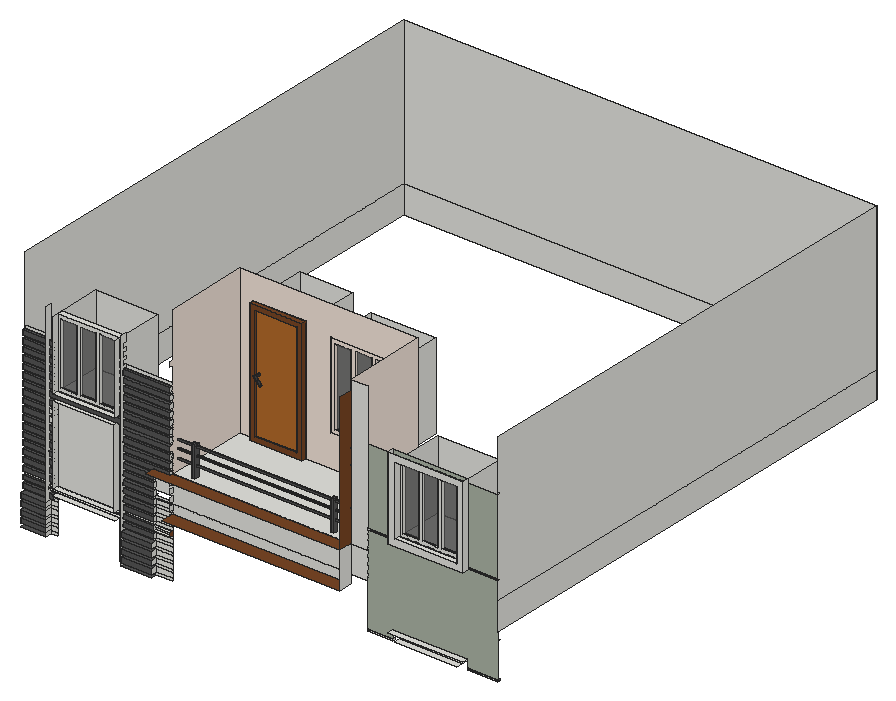
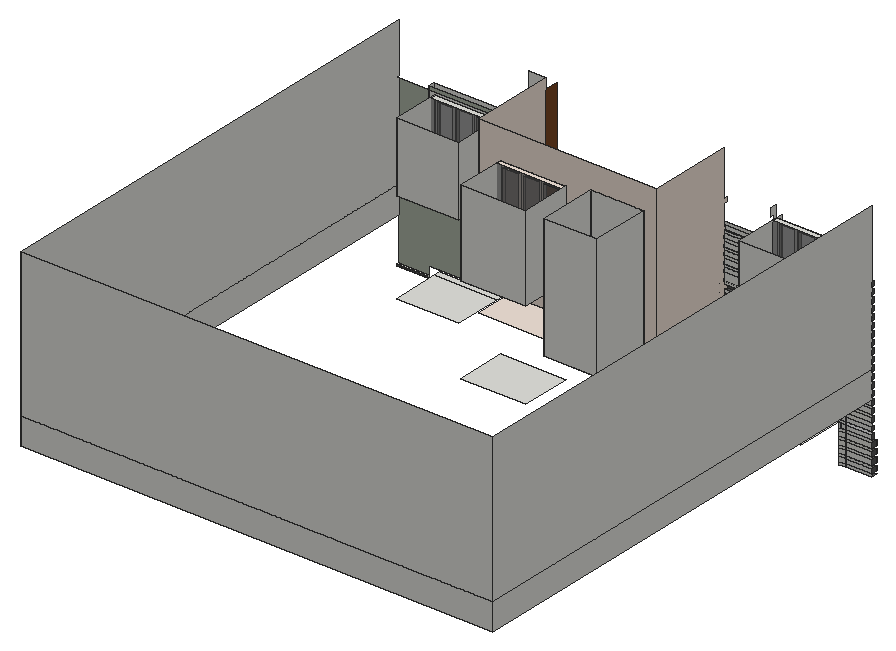
# SketchUp Ruby script. Lengths in inches.
U = 1.inch
M = Sketchup.active_model
def pt(a) = Geom::Point3d.new(a.map { |v| v * U })
def face(e, loops, mat)
  f = e.add_face(loops[0].map { |a| pt(a) })
  loops[1..].each { |l| e.add_face(l.map { |a| pt(a) }).erase! }
  f.material = f.back_material = mat if mat
  f
end
# faces: each face lists its corners as indices into pts; further lists are holes
def faces(e, pts, list, mat = nil) = list.each { |f| face(e, (f[0].is_a?(Array) ? f : [f]).map { |l| l.map { |i| pts[i] } }, mat) }
# xy, xz, yz: faces in a plane at the given z, y or x. An outline is a flat list of corners, or four numbers for a rectangle; further outlines are holes
def ring(l) = l.size == 4 ? [[l[0], l[1]], [l[2], l[1]], [l[2], l[3]], [l[0], l[3]]] : l.each_slice(2).to_a
def flat(e, list, mat, &to3) = list.each { |f| face(e, (f[0].is_a?(Array) ? f : [f]).map { |l| ring(l).map { |u, v| to3.(u, v) } }, mat) }
def xy(e, z, list, mat = nil) = flat(e, list, mat) { |x, y| [x, y, z] }
def xz(e, y, list, mat = nil) = flat(e, list, mat) { |x, z| [x, y, z] }
def yz(e, x, list, mat = nil) = flat(e, list, mat) { |y, z| [x, y, z] }
def lines(e, pts, list) = list.each { |a, b| e.add_line(pt(pts[a]), pt(pts[b])) }
# prism: a flat outline (further loops are holes) pulled along v
def prism(e, loops, v, mat = nil)
  f = face(e, loops, mat); d = Geom::Vector3d.new(v.map { |x| x * U })
  f.pushpull(f.normal.samedirection?(d) ? d.length : -d.length)
end
def box(e, o, s, mat = nil) = prism(e, [[o, [o[0] + s[0], o[1], o[2]], [o[0] + s[0], o[1] + s[1], o[2]], [o[0], o[1] + s[1], o[2]]]], [0, 0, s[2]], mat)
def at(x, y, z, deg = 0) = Geom::Transformation.translation(pt([x, y, z])) * Geom::Transformation.rotation(ORIGIN, Z_AXIS, deg.degrees)
def axes(o, x, y, z) = Geom::Transformation.new([*x, 0, *y, 0, *z, 0, *pt(o).to_a, 1])
def part(name) = M.definitions.add(name)
# library, detail: a bought-in or finely detailed component or shape, given as its bounding box
def library(name, o, s) = part(name).tap { |d| box(d.entities, o, s) }
def detail(e, o, s) = box(e.add_group.entities, o, s)
def put(e, d, t, mat = nil) = e.add_instance(d, t).tap { |i| i.material = mat if mat }
def group(e, t, mat = nil) = e.add_group.tap { |g| g.transformation = t; g.material = mat if mat }.entities
root = M.entities
M.materials.add("Generic\#1").color = [85, 85, 85]
M.materials.add("Generic\#2").color = [170, 178, 163]
M.materials.add("Generic\#4").color = [241, 227, 216]
M.materials.add("[Color M00]").color = [255, 255, 255]
M.materials.add("[Color M07]").color = [58, 58, 58]
M.materials.add("[Translucent Glass Gray]").color = [91, 91, 91]
M.materials["[Translucent Glass Gray]"].alpha = 0.55
M.materials.add("[Wood Bamboo]").color = [177, 105, 43]
M.materials.add("[Wood Veneer 01]").color = [120, 70, 37]
c1 = part("Group\#3")
xy(c1.entities,0,[[0,4.93,60.125,10.18]])
xy(c1.entities,5.66,[[5.66,4.93,54.46,7.18]],"[Wood Veneer 01]")
xy(c1.entities,68.44,[[8.18,1.47,8.18,7.18,9.93,7.18,9.93,2.62]],"[Color M07]")
xy(c1.entities,70.41,[[8.19,0,9.94,1.15,9.94,7.18,8.19,7.18]],"[Color M07]")
xy(c1.entities,134.78,[[5.66,4.93,54.46,7.18]])
xy(c1.entities,140.4375,[[0,4.93,60.125,10.18]],"[Wood Veneer 01]")
xz(c1.entities,4.93,[[[0,0,60.125,140.4375],[5.66,5.66,54.46,134.78]]],"[Wood Veneer 01]")
xz(c1.entities,7.18,[[[5.66,5.66,54.46,134.78],[8.18,68.44,8.19,70.41,9.94,70.41,9.93,68.44]],[8.18,68.44,8.19,70.41,9.94,70.41,9.93,68.44]],"[Wood Bamboo]")
xz(c1.entities,10.18,[[0,0,60.125,140.4375]])
yz(c1.entities,0,[[4.93,0,10.18,140.4375]],"[Wood Veneer 01]")
yz(c1.entities,5.66,[[4.93,5.66,7.18,134.78]],"[Wood Veneer 01]")
yz(c1.entities,54.46,[[4.93,5.66,7.18,134.78]],"[Wood Veneer 01]")
yz(c1.entities,60.125,[[4.93,0,10.18,140.4375]],"[Wood Veneer 01]")
p = [[8.19,0,70.41],[8.18,1.47,68.44],[14.45,1.47,61.21],[15.43,0,62.06],[15.45,2.62,62.07],[16.43,1.15,62.92],
  [9.93,2.62,68.44],[9.94,1.15,70.41],[8.19,7.18,70.41],[8.18,7.18,68.44],[9.93,7.18,68.44],[9.94,7.18,70.41],
  [8.95,0.93,69.83],[15.58,0.93,62.1875],[8.95,7.18,69.83]]
faces(c1.entities,p,[[0,1,2,3],[3,2,4,5],[1,6,4,2],[7,0,3,5],[6,7,5,4],[8,9,1,0],[10,11,7,6]],"[Color M07]")
lines(c1.entities,p,[[12,13],[14,12]])
c2 = part("Group\#1")
xy(c2.entities,0,[[0,0,70.8125,6.0625]])
xy(c2.entities,4.26,[[4.26,0,22.19,2.0625],[26.44,0,44.37,2.0625],[48.63,0,66.56,2.0625]])
xy(c2.entities,75.06,[[4.26,0,22.19,2.0625],[26.44,0,44.37,2.0625],[48.63,0,66.56,2.0625]])
xy(c2.entities,79.3125,[[0,0,70.8125,6.0625]])
xz(c2.entities,0,[[[0,0,70.8125,79.3125],[26.44,4.26,44.37,75.06],[4.26,4.26,22.19,75.06],[48.63,4.26,66.56,75.06]]])
xz(c2.entities,2.0625,[[4.26,4.26,22.19,75.06],[26.44,4.26,44.37,75.06],[48.63,4.26,66.56,75.06]],"[Translucent Glass Gray]")
xz(c2.entities,6.0625,[[0,0,70.8125,79.3125]],"[Translucent Glass Gray]")
yz(c2.entities,0,[[0,0,6.0625,79.3125]])
yz(c2.entities,4.26,[[0,4.26,2.0625,75.06]])
yz(c2.entities,22.19,[[0,4.26,2.0625,75.06]])
yz(c2.entities,26.44,[[0,4.26,2.0625,75.06]])
yz(c2.entities,44.37,[[0,4.26,2.0625,75.06]])
yz(c2.entities,48.63,[[0,4.26,2.0625,75.06]])
yz(c2.entities,66.56,[[0,4.26,2.0625,75.06]])
yz(c2.entities,70.8125,[[0,0,6.0625,79.3125]])
c3 = part("Group\#4")
xy(c3.entities,0,[[0,0,168,3.625]])
xy(c3.entities,5.375,[[0,0,168,3.625]])
xz(c3.entities,0,[[0,0,168,5.375]])
yz(c3.entities,0,[[0,0,3.625,5.375]])
c4 = part("Group\#2")
xy(c4.entities,0,[[0,0,74.5625,5.5]])
xy(c4.entities,4.83,[[4.83,0,23.24,2.5],[28.07,0,46.49,2.5],[51.32,0,69.73,2.5]])
xy(c4.entities,93.17,[[4.83,0,23.24,2.5],[28.07,0,46.49,2.5],[51.32,0,69.73,2.5]])
xy(c4.entities,98,[[0,0,74.5625,5.5]])
xz(c4.entities,0,[[[0,0,74.5625,98],[28.07,4.83,46.49,93.17],[51.32,4.83,69.73,93.17],[4.83,4.83,23.24,93.17]]])
xz(c4.entities,2.5,[[4.83,4.83,23.24,93.17],[28.07,4.83,46.49,93.17],[51.32,4.83,69.73,93.17]],"[Translucent Glass Gray]")
xz(c4.entities,5.5,[[0,0,74.5625,98]],"[Translucent Glass Gray]")
yz(c4.entities,0,[[0,0,5.5,98]])
yz(c4.entities,4.83,[[0,4.83,2.5,93.17]])
yz(c4.entities,23.24,[[0,4.83,2.5,93.17]])
yz(c4.entities,28.07,[[0,4.83,2.5,93.17]])
yz(c4.entities,46.49,[[0,4.83,2.5,93.17]])
yz(c4.entities,51.32,[[0,4.83,2.5,93.17]])
yz(c4.entities,69.73,[[0,4.83,2.5,93.17]])
yz(c4.entities,74.5625,[[0,0,5.5,98]])
xy(root,287.75,[[3.6875,24.0625,33.1875,31.0625],[118.35,24.0625,153.3125,31.0625]],"Generic\#1")
xy(root,291.0625,[[3.6875,24.0625,33.1875,31.0625],[118.35,24.0625,153.3125,31.0625]],"Generic\#1")
xy(root,296.4375,[[3.6875,24.0625,33.1875,31.0625],[118.35,24.0625,153.3125,31.0625]],"Generic\#1")
xy(root,299.75,[[3.6875,24.0625,33.1875,31.0625],[118.35,24.0625,153.3125,31.0625]],"Generic\#1")
xy(root,305.125,[[3.6875,24.0625,33.1875,31.0625],[118.35,24.0625,153.3125,31.0625]],"Generic\#1")
xy(root,308.4375,[[3.6875,24.0625,33.1875,31.0625],[118.35,24.0625,153.3125,31.0625]],"Generic\#1")
xy(root,313.8125,[[3.6875,24.0625,33.1875,31.0625],[118.35,24.0625,153.3125,31.0625]],"Generic\#1")
xy(root,315.5,[[395.4375,31.0625,423.8125,32.9375],[508.98,31.0625,543.6875,32.9375]])
xy(root,317.125,[[3.6875,24.0625,33.1875,31.0625],[118.35,24.0625,153.3125,31.0625]],"Generic\#1")
xy(root,317.5,[[395.4375,31.0625,423.8125,32.9375],[508.98,31.0625,543.6875,32.9375]])
xy(root,319.52,[[430.99,24.0625,501.8,31.0625],[430.99,31.0625,501.8,85.4375]])
xy(root,322.5,[[3.6875,24.0625,33.1875,31.0625],[118.35,24.0625,153.3125,31.0625]],"Generic\#1")
xy(root,325.8125,[[3.6875,27.4375,38.93,31.0625],[118.35,27.75,153.3125,31.0625]])
xy(root,326.69,[[423.8125,24.0625,508.98,31.0625]])
xy(root,331.1875,[[3.6875,27.4375,38.93,31.0625],[118.35,27.75,153.3125,31.0625]],"Generic\#1")
xy(root,331.7,[[40.36,24.0625,111.18,31.0625],[40.36,31.0625,111.18,85.4375]])
xy(root,333.91,[[275.98,127,350.54,183.625]])
xy(root,334.5,[[33.1875,27.75,118.35,31.0625],[153.3125,27.75,171.6875,31.0625]])
xy(root,334.5,[[3.6875,27.75,33.1875,31.0625],[118.35,27.75,153.3125,31.0625]],"Generic\#1")
xy(root,338.88,[[40.375,24.0625,110.67,31.0625],[33.1875,27.75,40.375,31.0625],[110.67,27.75,118.35,31.0625],[153.3125,27.75,171.6875,31.0625]])
xy(root,338.88,[[3.6875,27.75,33.1875,31.0625],[118.35,27.75,153.3125,31.0625]],"Generic\#1")
xy(root,339.3125,[[187.38,127,247.51,193.75]])
xy(root,343.1875,[[3.6875,27.4375,39.4375,31.0625],[118.35,27.4375,153.3125,31.0625]],"Generic\#1")
xy(root,348.5625,[[3.6875,27.4375,39.4375,31.0625],[118.35,27.4375,153.3125,31.0625]],"Generic\#1")
xy(root,351.875,[[3.6875,27.4375,39.4375,31.0625],[118.35,27.4375,153.3125,31.0625]],"Generic\#1")
xy(root,356.125,[[171.6875,15.8125,375.6875,31.0625]],"[Wood Veneer 01]")
xy(root,357.25,[[3.6875,27.4375,39.4375,31.0625],[118.35,27.4375,153.3125,31.0625]],"Generic\#1")
xy(root,360.5625,[[3.6875,27.4375,39.4375,31.0625],[118.35,27.4375,153.3125,31.0625]],"Generic\#1")
xy(root,365.9375,[[3.6875,27.4375,39.4375,31.0625],[118.35,27.4375,153.3125,31.0625]],"Generic\#1")
xy(root,366.875,[[171.6875,31.0625,375.6875,127]],"Generic\#4")
xy(root,369.25,[[3.6875,27.4375,39.4375,31.0625],[118.35,27.4375,153.3125,31.0625]],"Generic\#1")
xy(root,374.625,[[3.6875,27.4375,39.4375,31.0625],[118.35,27.4375,153.3125,31.0625]],"Generic\#1")
xy(root,377.9375,[[3.6875,27.4375,39.4375,31.0625],[118.35,27.4375,153.3125,31.0625]],"Generic\#1")
xy(root,383.3125,[[3.6875,27.4375,39.4375,31.0625],[118.35,27.4375,153.3125,31.0625]],"Generic\#1")
xy(root,386.625,[[3.6875,27.4375,39.4375,31.0625],[118.35,27.4375,153.3125,31.0625]],"Generic\#1")
xy(root,392,[[3.6875,27.4375,39.4375,31.0625],[118.35,27.4375,153.3125,31.0625]],"Generic\#1")
xy(root,395.3125,[[3.6875,27.4375,39.4375,31.0625],[118.35,27.4375,153.3125,31.0625]],"Generic\#1")
xy(root,397.75,[[153.3125,27.4375,171.6875,31.0625],[[171.6875,31.0625,171.6875,127,187.38,127,187.38,193.75,247.51,193.75,247.51,127,375.6875,127,375.6875,31.0625],[190.01,36.375,193.64,40.875],[348.74,36.375,352.11,40.5625]],[190.01,36.375,193.64,40.875],[348.74,36.375,352.11,40.5625]])
xy(root,397.75,[[153.3125,15.8125,375.6875,15.8125,375.6875,31.0625,171.6875,31.0625,171.6875,27.4375,153.3125,27.4375]],"[Wood Veneer 01]")
xy(root,400.6875,[[3.6875,27.4375,39.4375,31.0625],[118.35,27.4375,171.6875,31.0625]],"Generic\#1")
xy(root,404,[[33.1875,27.4375,39.4375,31.0625]])
xy(root,404,[[3.6875,27.4375,33.1875,31.0625],[118.35,27.4375,171.6875,31.0625]],"Generic\#1")
xy(root,409.375,[[3.6875,27.4375,33.1875,31.0625],[118.35,27.4375,171.6875,31.0625]],"Generic\#1")
xy(root,410.15,[[171.6875,37.35,375.6875,39.16]],"Generic\#1")
xy(root,411.78,[[171.6875,37.35,375.6875,39.16]],"Generic\#1")
xy(root,412.6875,[[3.6875,27.4375,33.1875,31.0625],[118.35,27.4375,171.6875,31.0625]],"Generic\#1")
xy(root,417.46,[[423.8125,24.0625,508.98,31.0625]])
xy(root,418.0625,[[3.6875,27.4375,33.1875,31.0625],[118.35,27.4375,171.6875,31.0625]],"Generic\#1")
xy(root,418.375,[[395.4375,31.0625,423.8125,32.9375],[508.98,31.0625,543.6875,32.9375]])
xy(root,419.875,[[171.6875,37.34,375.6875,39.15]],"Generic\#1")
xy(root,420.375,[[395.4375,31.0625,423.8125,32.9375],[508.98,31.0625,543.6875,32.9375]])
xy(root,421.375,[[3.6875,27.4375,39.4375,31.0625],[118.35,27.4375,171.6875,31.0625]],"Generic\#1")
xy(root,421.5,[[171.6875,37.34,375.6875,39.15]],"Generic\#1")
xy(root,424.64,[[430.99,24.0625,501.8,31.0625],[430.99,31.0625,501.8,85.4375]])
xy(root,426.75,[[3.6875,27.4375,39.4375,31.0625],[118.35,27.4375,171.6875,31.0625]],"Generic\#1")
xy(root,429.03,[[40.375,24.0625,110.67,31.0625]])
xy(root,429.65,[[171.6875,37.35,375.6875,39.16]],"Generic\#1")
xy(root,431.28,[[190.01,39.16,193.64,40.875],[348.74,39.16,352.11,40.5625]])
xy(root,431.28,[[171.6875,37.35,190.01,39.16],[193.64,37.35,348.74,39.16],[352.11,37.35,375.6875,39.16]],"Generic\#1")
xy(root,432.78,[[190.01,36.375,193.64,40.875],[348.74,36.375,352.11,40.5625]],"Generic\#1")
xy(root,434.04,[[275.98,127,350.54,183.625]])
xy(root,436.2,[[40.36,24.0625,111.18,31.0625],[40.36,31.0625,111.18,85.4375]])
xy(root,438.75,[[3.6875,27.4375,39.68,31.0625],[118.35,27.4375,171.6875,31.0625]],"Generic\#1")
xy(root,444.125,[[3.6875,27.4375,39.68,31.0625],[118.35,27.4375,171.6875,31.0625]],"Generic\#1")
xy(root,447.4375,[[3.6875,27.4375,39.68,31.0625],[118.35,27.4375,171.6875,31.0625]],"Generic\#1")
xy(root,452.8125,[[3.6875,27.4375,39.68,31.0625],[118.35,27.4375,171.6875,31.0625]],"Generic\#1")
xy(root,456.125,[[3.6875,27.4375,39.68,31.0625],[118.35,27.4375,171.6875,31.0625]],"Generic\#1")
xy(root,461.5,[[3.6875,27.4375,39.68,31.0625],[118.35,27.4375,171.6875,31.0625]],"Generic\#1")
xy(root,464.8125,[[3.6875,27.4375,39.68,31.0625],[118.35,27.4375,171.6875,31.0625]],"Generic\#1")
xy(root,470.1875,[[3.6875,27.4375,39.68,31.0625],[118.35,27.4375,171.6875,31.0625]],"Generic\#1")
xy(root,473.5,[[3.6875,27.4375,39.68,31.0625],[118.35,27.4375,171.6875,31.0625]],"Generic\#1")
xy(root,478.875,[[3.6875,27.4375,39.68,31.0625],[118.35,27.4375,171.6875,31.0625]],"Generic\#1")
xy(root,482.1875,[[118.35,26.9375,171.6875,30.5625],[3.6875,27.4375,39.68,31.0625],[118.35,30.5625,171.6875,31.0625]],"Generic\#1")
xy(root,487.5625,[[118.35,26.9375,171.6875,30.5625],[3.6875,27.4375,39.68,31.0625],[118.35,30.5625,171.6875,31.0625]],"Generic\#1")
xz(root,24.0625,[[[423.8125,417.46,508.98,511.13],[430.99,424.64,501.8,503.95]]])
xz(root,24.0625,[[3.6875,291.0625,33.1875,296.4375],[118.35,291.0625,153.3125,296.4375],[3.6875,299.75,33.1875,305.125],[118.35,299.75,153.3125,305.125],[3.6875,308.4375,33.1875,313.8125],
  [118.35,308.4375,153.3125,313.8125],[3.6875,317.125,33.1875,322.5],[118.35,317.125,153.3125,322.5]],"Generic\#1")
xz(root,26.9375,[[118.35,482.1875,171.6875,487.5625]],"Generic\#1")
xz(root,27.4375,[[33.1875,404,39.4375,409.375],[33.1875,412.6875,38.875,418.0625]])
xz(root,27.4375,[[3.6875,325.8125,38.93,331.1875],[3.6875,343.1875,39.4375,348.5625],[118.35,343.1875,153.3125,348.5625],[3.6875,351.875,39.4375,357.25],[118.35,351.875,153.3125,357.25],
  [3.6875,360.5625,39.4375,365.9375],[118.35,360.5625,153.3125,365.9375],[3.6875,369.25,39.4375,374.625],[118.35,369.25,153.3125,374.625],[3.6875,377.9375,39.4375,383.3125],
  [118.35,377.9375,153.3125,383.3125],[3.6875,386.625,39.4375,392],[118.35,386.625,153.3125,392],[3.6875,395.3125,39.4375,400.6875],[118.35,395.3125,153.3125,395.3125,153.3125,397.75,171.6875,397.75,171.6875,400.6875,118.35,400.6875],
  [3.6875,404,33.1875,409.375],[118.35,404,171.6875,409.375],[3.6875,412.6875,33.1875,418.0625],[118.35,412.6875,171.6875,418.0625],[3.6875,421.375,39.4375,426.75],
  [118.35,421.375,171.6875,426.75],[3.6875,438.75,39.68,444.125],[118.35,438.75,171.6875,444.125],[3.6875,447.4375,39.68,452.8125],[118.35,447.4375,171.6875,452.8125],
  [3.6875,456.125,39.68,461.5],[118.35,456.125,171.6875,461.5],[3.6875,464.8125,39.68,470.1875],[118.35,464.8125,171.6875,470.1875],[3.6875,473.5,39.68,478.875],
  [118.35,473.5,171.6875,478.875],[3.6875,482.1875,39.68,487.5625]],"Generic\#1")
xz(root,27.75,[[118.35,325.8125,153.3125,331.1875],[3.6875,334.5,33.1875,338.88],[118.35,334.5,153.3125,338.88]],"Generic\#1")
xz(root,30.5625,[[118.35,482.1875,171.6875,487.5625]])
xz(root,31.0625,[[3.6875,287.75,33.1875,291.0625],[33.1875,287.75,40.36,291.0625],[111.18,287.75,118.35,291.0625],[118.35,287.75,153.3125,291.0625],[153.3125,287.75,171.6875,291.0625],
  [3.6875,291.0625,33.1875,296.4375],[33.1875,291.0625,40.36,296.4375],[111.18,291.0625,118.35,296.4375],[153.3125,291.0625,171.6875,296.4375],[3.6875,296.4375,33.1875,299.75],
  [33.1875,296.4375,40.36,299.75],[111.18,296.4375,118.35,299.75],[118.35,296.4375,153.3125,299.75],[153.3125,296.4375,171.6875,299.75],[3.6875,299.75,33.1875,305.125],
  [33.1875,299.75,40.36,305.125],[111.18,299.75,118.35,305.125],[153.3125,299.75,171.6875,305.125],[3.6875,305.125,33.1875,308.4375],[33.1875,305.125,40.36,308.4375],
  [111.18,305.125,118.35,308.4375],[118.35,305.125,153.3125,308.4375],[153.3125,305.125,171.6875,308.4375],[3.6875,308.4375,33.1875,313.8125],[33.1875,308.4375,40.36,313.8125],
  [111.18,308.4375,118.35,313.8125],[153.3125,308.4375,171.6875,313.8125],[3.6875,313.8125,33.1875,317.125],[33.1875,313.8125,40.36,317.125],[111.18,313.8125,118.35,317.125],
  [118.35,313.8125,153.3125,317.125],[153.3125,313.8125,171.6875,317.125],[3.6875,317.125,33.1875,322.5],[33.1875,317.125,40.36,322.5],[111.18,317.125,118.35,322.5],
  [153.3125,317.125,171.6875,322.5],[3.6875,322.5,33.1875,325.8125],[33.1875,322.5,40.36,325.8125],[111.18,322.5,118.35,325.8125],[118.35,322.5,153.3125,325.8125],
  [153.3125,322.5,171.6875,325.8125],[3.6875,325.8125,33.1875,331.1875],[33.1875,325.8125,38.93,331.1875],[38.93,325.8125,40.36,331.1875],[111.18,325.8125,118.35,331.1875],
  [118.35,325.8125,153.3125,331.1875],[153.3125,325.8125,171.6875,331.1875],[33.1875,331.1875,33.1875,334.5,118.35,334.5,118.35,331.1875,111.18,331.1875,111.18,331.7,40.36,331.7,40.36,331.1875],[118.35,331.1875,153.3125,334.5],[153.3125,331.1875,171.6875,334.5],
  [3.6875,334.5,33.1875,338.88],[33.1875,334.5,118.35,338.88],[153.3125,334.5,171.6875,338.88],[3.6875,338.88,33.1875,343.1875],[33.1875,338.88,40.375,343.1875],
  [40.375,338.88,110.67,429.03],[110.67,338.88,118.35,343.1875],[118.35,338.88,153.3125,343.1875],[153.3125,338.88,171.6875,343.1875],[3.6875,343.1875,33.1875,348.5625],
  [33.1875,343.1875,39.4375,348.5625],[39.4375,343.1875,40.375,348.5625],[110.67,343.1875,118.35,348.5625],[118.35,343.1875,153.3125,348.5625],[153.3125,343.1875,171.6875,348.5625],
  [3.6875,348.5625,33.1875,351.875],[33.1875,348.5625,40.375,351.875],[110.67,348.5625,118.35,351.875],[118.35,348.5625,153.3125,351.875],[153.3125,348.5625,171.6875,351.875],
  [3.6875,351.875,33.1875,357.25],[33.1875,351.875,39.4375,357.25],[39.4375,351.875,40.375,357.25],[110.67,351.875,118.35,357.25],[118.35,351.875,153.3125,357.25],
  [153.3125,351.875,171.6875,357.25],[171.6875,356.125,375.6875,366.875],[3.6875,357.25,33.1875,360.5625],[33.1875,357.25,40.375,360.5625],[110.67,357.25,118.35,360.5625],
  [118.35,357.25,153.3125,360.5625],[153.3125,357.25,171.6875,360.5625],[3.6875,360.5625,33.1875,365.9375],[33.1875,360.5625,39.4375,365.9375],[39.4375,360.5625,40.375,365.9375],
  [110.67,360.5625,118.35,365.9375],[118.35,360.5625,153.3125,365.9375],[153.3125,360.5625,171.6875,365.9375],[3.6875,365.9375,33.1875,369.25],[33.1875,365.9375,40.375,369.25],
  [110.67,365.9375,118.35,369.25],[118.35,365.9375,153.3125,369.25],[153.3125,365.9375,171.6875,366.875],[153.3125,366.875,375.6875,366.875,375.6875,397.75,171.6875,397.75,171.6875,395.3125,153.3125,395.3125,153.3125,374.625,171.6875,374.625,171.6875,369.25,153.3125,369.25],[375.6875,366.875,395.4375,397.75],
  [3.6875,369.25,33.1875,374.625],[33.1875,369.25,39.4375,374.625],[39.4375,369.25,40.375,374.625],[110.67,369.25,118.35,374.625],[118.35,369.25,153.3125,374.625],
  [3.6875,374.625,33.1875,377.9375],[33.1875,374.625,40.375,377.9375],[110.67,374.625,118.35,377.9375],[118.35,374.625,153.3125,377.9375],[3.6875,377.9375,33.1875,383.3125],
  [33.1875,377.9375,39.4375,383.3125],[39.4375,377.9375,40.375,383.3125],[110.67,377.9375,118.35,383.3125],[118.35,377.9375,153.3125,383.3125],[3.6875,383.3125,33.1875,386.625],
  [33.1875,383.3125,40.375,386.625],[110.67,383.3125,118.35,386.625],[118.35,383.3125,153.3125,386.625],[3.6875,386.625,33.1875,392],[33.1875,386.625,39.4375,392],
  [39.4375,386.625,40.375,392],[110.67,386.625,118.35,392],[118.35,386.625,153.3125,392],[3.6875,392,33.1875,395.3125],[33.1875,392,40.375,395.3125],
  [110.67,392,118.35,395.3125],[118.35,392,153.3125,395.3125],[3.6875,395.3125,33.1875,400.6875],[33.1875,395.3125,39.4375,400.6875],[39.4375,395.3125,40.375,400.6875],
  [110.67,395.3125,118.35,400.6875],[118.35,395.3125,118.35,400.6875,171.6875,400.6875,171.6875,397.75,153.3125,397.75,153.3125,395.3125],[375.6875,397.75,395.4375,565.75],[3.6875,400.6875,33.1875,404],[33.1875,400.6875,40.375,404],
  [110.67,400.6875,118.35,404],[118.35,400.6875,171.6875,404],[3.6875,404,33.1875,409.375],[33.1875,404,39.4375,409.375],[39.4375,404,40.375,409.375],
  [118.35,404,171.6875,409.375],[3.6875,409.375,33.1875,412.6875],[33.1875,409.375,40.375,412.6875],[110.67,409.375,118.35,412.6875],[118.35,409.375,171.6875,412.6875],
  [3.6875,412.6875,33.1875,418.0625],[33.1875,412.6875,40.375,418.0625],[110.67,412.6875,118.35,418.0625],[118.35,412.6875,171.6875,418.0625],[423.8125,417.46,508.98,418.375],
  [3.6875,418.0625,33.1875,421.375],[33.1875,418.0625,40.375,421.375],[110.67,418.0625,118.35,421.375],[118.35,418.0625,171.6875,421.375],[423.8125,418.375,508.98,420.375],
  [[423.8125,420.375,508.98,507.02],[430.99,424.64,501.8,503.95]],[3.6875,421.375,33.1875,426.75],[33.1875,421.375,39.4375,426.75],[39.4375,421.375,40.375,426.75],[3.6875,426.75,33.1875,438.75],
  [33.1875,426.75,40.375,429.03],[110.67,426.75,118.35,429.03],[118.35,426.75,171.6875,438.75],[33.1875,429.03,33.1875,438.75,40.36,438.75,40.36,436.2,111.18,436.2,111.18,438.75,118.35,438.75,118.35,429.03],[3.6875,438.75,33.1875,444.125],
  [33.1875,438.75,39.68,444.125],[39.68,438.75,40.36,444.125],[111.18,438.75,118.35,444.125],[118.35,438.75,171.6875,444.125],[3.6875,444.125,33.1875,447.4375],
  [33.1875,444.125,40.36,447.4375],[111.18,444.125,118.35,447.4375],[118.35,444.125,171.6875,447.4375],[3.6875,447.4375,33.1875,452.8125],[33.1875,447.4375,39.68,452.8125],
  [39.68,447.4375,40.36,452.8125],[111.18,447.4375,118.35,452.8125],[118.35,447.4375,171.6875,452.8125],[3.6875,452.8125,33.1875,456.125],[33.1875,452.8125,40.36,456.125],
  [111.18,452.8125,118.35,456.125],[118.35,452.8125,171.6875,456.125],[3.6875,456.125,33.1875,461.5],[33.1875,456.125,39.68,461.5],[39.68,456.125,40.36,461.5],
  [111.18,456.125,118.35,461.5],[118.35,456.125,171.6875,461.5],[3.6875,461.5,33.1875,464.8125],[33.1875,461.5,40.36,464.8125],[111.18,461.5,118.35,464.8125],
  [118.35,461.5,171.6875,464.8125],[3.6875,464.8125,33.1875,470.1875],[33.1875,464.8125,39.68,470.1875],[39.68,464.8125,40.36,470.1875],[111.18,464.8125,118.35,470.1875],
  [118.35,464.8125,171.6875,470.1875],[3.6875,470.1875,33.1875,473.5],[33.1875,470.1875,40.36,473.5],[111.18,470.1875,118.35,473.5],[118.35,470.1875,171.6875,473.5],
  [3.6875,473.5,33.1875,478.875],[33.1875,473.5,39.68,478.875],[39.68,473.5,40.36,478.875],[111.18,473.5,118.35,478.875],[118.35,473.5,171.6875,478.875],
  [3.6875,478.875,33.1875,482.1875],[33.1875,478.875,40.36,482.1875],[111.18,478.875,118.35,482.1875],[118.35,478.875,171.6875,482.1875],[3.6875,482.1875,33.1875,487.5625],
  [33.1875,482.1875,39.68,487.5625],[39.68,482.1875,40.36,487.5625],[111.18,482.1875,118.35,487.5625],[3.6875,487.5625,33.1875,490.875],[33.1875,487.5625,40.36,490.875],
  [111.18,487.5625,118.35,490.875],[118.35,487.5625,171.6875,490.875]])
xz(root,31.0625,[[395.4375,317.5,423.8125,317.5,423.8125,326.69,508.98,326.69,508.98,317.5,543.6875,317.5,543.6875,418.375,508.98,418.375,508.98,417.46,423.8125,417.46,423.8125,418.375,395.4375,418.375],[395.4375,420.375,423.8125,420.375,423.8125,511.13,508.98,511.13,508.98,420.375,543.6875,420.375,543.6875,507.02,395.4375,507.02]],"Generic\#2")
xz(root,31.0625,[[3.6875,331.1875,33.1875,334.5]],"[Color M00]")
xz(root,32.9375,[[395.4375,315.5,423.8125,317.5],[508.98,315.5,543.6875,317.5],[395.4375,418.375,423.8125,420.375],[508.98,418.375,543.6875,420.375]],"Generic\#1")
xz(root,36.375,[[190.01,397.75,193.64,432.78],[348.74,397.75,352.11,432.78]],"Generic\#1")
xz(root,37.34,[[171.6875,419.875,375.6875,421.5]],"Generic\#1")
xz(root,37.35,[[171.6875,410.15,375.6875,411.78],[171.6875,429.65,375.6875,431.28]],"Generic\#1")
xz(root,39.15,[[171.6875,419.875,375.6875,421.5]])
xz(root,39.16,[[171.6875,410.15,375.6875,411.78],[171.6875,429.65,375.6875,431.28]])
xz(root,40.5625,[[348.74,397.75,352.11,431.28],[348.74,431.28,352.11,432.78]])
xz(root,40.875,[[190.01,397.75,193.64,431.28],[190.01,431.28,193.64,432.78]])
xz(root,85.4375,[[430.99,424.64,501.8,503.95],[40.36,436.2,111.18,515.52]])
xz(root,127,[[[171.6875,397.75,187.38,397.75,187.38,538.1875,247.51,538.1875,247.51,397.75,375.6875,397.75,375.6875,565.75,171.6875,565.75],[275.98,434.04,350.54,532.04]]],"Generic\#4")
xz(root,183.625,[[275.98,434.04,350.54,532.04]])
xz(root,193.75,[[187.38,397.75,247.51,538.1875]])
xz(root,571.0625,[[3.6875,366.875,543.6875,397.75],[3.6875,397.75,543.6875,565.75]])
yz(root,3.6875,[[31.0625,366.875,571.0625,397.75],[31.0625,397.75,571.0625,565.75]])
yz(root,3.6875,[[24.0625,291.0625,31.0625,296.4375],[24.0625,299.75,31.0625,305.125],[24.0625,308.4375,31.0625,313.8125],[24.0625,317.125,31.0625,322.5],[27.4375,325.8125,31.0625,331.1875],
  [27.75,334.5,31.0625,338.88],[27.4375,343.1875,31.0625,348.5625],[27.4375,351.875,31.0625,357.25],[27.4375,360.5625,31.0625,365.9375],[27.4375,369.25,31.0625,374.625],
  [27.4375,377.9375,31.0625,383.3125],[27.4375,386.625,31.0625,392],[27.4375,395.3125,31.0625,400.6875],[27.4375,404,31.0625,409.375],[27.4375,412.6875,31.0625,418.0625],
  [27.4375,421.375,31.0625,426.75],[27.4375,438.75,31.0625,444.125],[27.4375,447.4375,31.0625,452.8125],[27.4375,456.125,31.0625,461.5],[27.4375,464.8125,31.0625,470.1875],
  [27.4375,473.5,31.0625,478.875],[27.4375,482.1875,31.0625,487.5625]],"Generic\#1")
yz(root,33.1875,[[24.0625,287.75,31.0625,291.0625],[24.0625,291.0625,31.0625,296.4375],[24.0625,296.4375,31.0625,299.75],[24.0625,299.75,31.0625,305.125],[24.0625,305.125,31.0625,308.4375],
  [24.0625,308.4375,31.0625,313.8125],[24.0625,313.8125,31.0625,317.125],[24.0625,317.125,31.0625,322.5],[24.0625,322.5,24.0625,522.69,31.0625,522.69,31.0625,418.0625,27.4375,418.0625,27.4375,412.6875,31.0625,412.6875,31.0625,409.375,27.4375,409.375,27.4375,404,31.0625,404,31.0625,338.88,27.75,338.88,27.75,334.5,31.0625,334.5,31.0625,322.5],[27.75,334.5,31.0625,338.88],
  [27.4375,404,31.0625,409.375],[27.4375,412.6875,31.0625,418.0625]])
yz(root,38.875,[[27.4375,412.6875,30.4375,418.0625]])
yz(root,38.93,[[27.4375,325.8125,31.0625,331.1875]])
yz(root,39.4375,[[27.4375,343.1875,31.0625,348.5625],[27.4375,351.875,31.0625,357.25],[27.4375,360.5625,31.0625,365.9375],[27.4375,369.25,31.0625,374.625],[27.4375,377.9375,31.0625,383.3125],
  [27.4375,386.625,31.0625,392],[27.4375,395.3125,31.0625,400.6875],[27.4375,421.375,31.0625,426.75]])
yz(root,39.68,[[27.4375,438.75,31.0625,444.125],[27.4375,447.4375,31.0625,452.8125],[27.4375,456.125,31.0625,461.5],[27.4375,464.8125,31.0625,470.1875],[27.4375,473.5,31.0625,478.875],
  [27.4375,482.1875,31.0625,487.5625]])
yz(root,40.36,[[24.0625,436.2,31.0625,515.52],[31.0625,436.2,85.4375,515.52]])
yz(root,40.375,[[24.0625,338.88,31.0625,429.03]])
yz(root,110.67,[[24.0625,338.88,31.0625,429.03]])
yz(root,111.18,[[24.0625,436.2,31.0625,515.52],[31.0625,436.2,85.4375,515.52]])
yz(root,118.35,[[24.0625,287.75,31.0625,291.0625],[24.0625,291.0625,31.0625,296.4375],[24.0625,296.4375,31.0625,299.75],[24.0625,299.75,31.0625,305.125],[24.0625,305.125,31.0625,308.4375],
  [24.0625,308.4375,31.0625,313.8125],[24.0625,313.8125,31.0625,317.125],[24.0625,317.125,31.0625,322.5],[24.0625,322.5,31.0625,322.5,31.0625,325.8125,27.75,325.8125,27.75,331.1875,31.0625,331.1875,31.0625,334.5,27.75,334.5,27.75,338.88,31.0625,338.88,31.0625,343.1875,27.4375,343.1875,27.4375,348.5625,31.0625,348.5625,31.0625,351.875,27.4375,351.875,27.4375,357.25,31.0625,357.25,31.0625,360.5625,27.4375,360.5625,27.4375,365.9375,31.0625,365.9375,31.0625,369.25,27.4375,369.25,27.4375,374.625,31.0625,374.625,31.0625,377.9375,27.4375,377.9375,27.4375,383.3125,31.0625,383.3125,31.0625,386.625,27.4375,386.625,27.4375,392,31.0625,392,31.0625,395.3125,27.4375,395.3125,27.4375,400.6875,31.0625,400.6875,31.0625,404,27.4375,404,27.4375,409.375,31.0625,409.375,31.0625,412.6875,27.4375,412.6875,27.4375,418.0625,31.0625,418.0625,31.0625,421.375,27.4375,421.375,27.4375,426.75,31.0625,426.75,31.0625,438.75,27.4375,438.75,27.4375,444.125,31.0625,444.125,31.0625,447.4375,27.4375,447.4375,27.4375,452.8125,31.0625,452.8125,31.0625,456.125,27.4375,456.125,27.4375,461.5,31.0625,461.5,31.0625,464.8125,27.4375,464.8125,27.4375,470.1875,31.0625,470.1875,31.0625,473.5,27.4375,473.5,27.4375,478.875,31.0625,478.875,31.0625,482.1875,26.9375,482.1875,26.9375,487.5625,31.0625,487.5625,31.0625,490.875,26.9375,490.875,26.9375,496.25,31.0625,496.25,31.0625,499.5625,27,499.5625,27,504.9375,31.0625,504.9375,31.0625,508.25,27,508.25,27,513.625,31.0625,513.625,31.0625,522.69,24.0625,522.69],[27.75,325.8125,31.0625,331.1875],
  [27.75,334.5,31.0625,338.88],[27.4375,343.1875,31.0625,348.5625],[27.4375,351.875,31.0625,357.25],[27.4375,360.5625,31.0625,365.9375],[27.4375,369.25,31.0625,374.625],
  [27.4375,377.9375,31.0625,383.3125],[27.4375,386.625,31.0625,392],[27.4375,395.3125,31.0625,400.6875],[27.4375,404,31.0625,409.375],[27.4375,412.6875,31.0625,418.0625],
  [27.4375,438.75,31.0625,444.125],[27.4375,447.4375,31.0625,452.8125],[27.4375,456.125,31.0625,461.5],[27.4375,464.8125,31.0625,470.1875],[27.4375,473.5,31.0625,478.875],
  [26.9375,482.1875,30.5625,487.5625],[30.5625,482.1875,31.0625,487.5625]])
yz(root,153.3125,[[24.0625,291.0625,31.0625,296.4375],[24.0625,299.75,31.0625,305.125],[24.0625,308.4375,31.0625,313.8125],[24.0625,317.125,31.0625,322.5],[27.75,325.8125,31.0625,331.1875],
  [27.75,334.5,31.0625,338.88],[27.4375,343.1875,31.0625,348.5625],[27.4375,351.875,31.0625,357.25],[27.4375,360.5625,31.0625,365.9375],[27.4375,369.25,31.0625,374.625],
  [27.4375,377.9375,31.0625,383.3125],[27.4375,386.625,31.0625,392],[27.4375,395.3125,31.0625,397.75]])
yz(root,171.6875,[[27.4375,356.125,31.0625,357.25],[27.4375,360.5625,31.0625,365.9375],[27.4375,369.25,31.0625,374.625],[27.4375,377.9375,31.0625,383.3125],[27.4375,386.625,31.0625,392],
  [27.4375,395.3125,31.0625,397.75],[27.4375,397.75,31.0625,400.6875],[27.4375,404,31.0625,409.375],[27.4375,412.6875,30.4375,418.0625],[30.4375,412.6875,31.0625,418.0625],
  [27.4375,430.0625,31.0625,435.4375],[27.4375,438.75,31.0625,444.125],[27.4375,447.4375,31.0625,452.8125],[27.4375,456.125,31.0625,461.5],[27.4375,464.8125,31.0625,470.1875],
  [27.4375,473.5,31.0625,478.875],[26.9375,482.1875,30.5625,487.5625]])
yz(root,171.6875,[[[31.0625,397.75,127,397.75,127,565.75,31.0625,565.75,31.0625,513.625,27,513.625,27,508.25,31.0625,508.25,31.0625,487.5625,30.5625,487.5625,30.5625,482.1875,31.0625,482.1875,31.0625,426.75,27.4375,426.75,27.4375,421.375,31.0625,421.375],[37.35,410.15,39.16,411.78],[37.34,419.875,39.15,421.5],[37.35,429.65,39.16,431.28]]],"Generic\#4")
yz(root,171.6875,[[27.75,334.5,31.0625,338.88]],"[Wood Veneer 01]")
yz(root,187.38,[[127,397.75,193.75,538.1875]])
yz(root,190.01,[[36.375,397.75,40.875,431.28],[36.375,431.28,37.35,432.78],[37.35,431.28,39.16,432.78],[39.16,431.28,40.875,432.78]],"Generic\#1")
yz(root,193.64,[[36.375,397.75,40.875,431.28],[36.375,431.28,37.35,432.78],[37.35,431.28,39.16,432.78],[39.16,431.28,40.875,432.78]],"Generic\#1")
yz(root,247.51,[[127,397.75,193.75,538.1875]])
yz(root,275.98,[[127,434.04,183.625,532.04]])
yz(root,348.74,[[36.375,397.75,40.5625,431.28],[36.375,431.28,37.35,432.78],[37.35,431.28,39.16,432.78],[39.16,431.28,40.5625,432.78]],"Generic\#1")
yz(root,350.54,[[127,434.04,183.625,532.04]])
yz(root,352.11,[[36.375,397.75,40.5625,431.28],[36.375,431.28,37.35,432.78],[37.35,431.28,39.16,432.78],[39.16,431.28,40.5625,432.78]],"Generic\#1")
yz(root,375.6875,[[15.8125,356.125,31.0625,397.75]])
yz(root,375.6875,[[[31.0625,397.75,127,565.75],[37.35,410.15,39.16,411.78],[37.34,419.875,39.15,421.5],[37.35,429.65,39.16,431.28]]],"Generic\#4")
yz(root,375.6875,[[15.8125,397.75,31.0625,554.25]],"[Wood Veneer 01]")
yz(root,395.4375,[[31.0625,315.5,32.9375,317.5],[31.0625,418.375,32.9375,420.375]])
yz(root,423.8125,[[31.0625,315.5,32.9375,317.5],[24.0625,417.46,31.0625,511.13],[31.0625,418.375,32.9375,420.375]])
yz(root,430.99,[[24.0625,424.64,31.0625,503.95],[31.0625,424.64,85.4375,503.95]])
yz(root,501.8,[[24.0625,424.64,31.0625,503.95],[31.0625,424.64,85.4375,503.95]])
yz(root,508.98,[[31.0625,315.5,32.9375,317.5],[24.0625,417.46,31.0625,511.13],[31.0625,418.375,32.9375,420.375]])
yz(root,543.6875,[[31.0625,366.875,571.0625,397.75],[31.0625,397.75,571.0625,397.75,571.0625,565.75,31.0625,565.75,31.0625,509.02,32.9375,509.02,32.9375,507.02,31.0625,507.02,31.0625,420.375,32.9375,420.375,32.9375,418.375,31.0625,418.375]])
p = [[171.6875,38.07,411.05],[191.78,38.07,411.05],[171.6875,38.07,420.73],[191.78,38.07,420.73],[171.6875,38.07,430.42],[191.78,38.07,430.42],
  [349.97,38.07,430.42],[375.6875,38.07,430.42],[349.97,38.07,420.73],[349.97,38.07,411.05],[375.6875,38.07,411.05],[375.6875,38.07,420.73],
  [349.97,38.07,397.75],[191.78,38.07,397.75],[38.93,27.4375,325.8125],[40.36,27.4375,325.8125],[39.4375,27.4375,426.75],[40.375,27.4375,426.75],
  [39.4375,27.4375,421.375],[40.375,27.4375,421.375],[39.4375,27.4375,400.6875],[40.375,27.4375,400.6875],[39.4375,27.4375,386.625],[40.375,27.4375,386.625],
  [39.4375,27.4375,377.9375],[40.375,27.4375,377.9375],[39.4375,27.4375,374.625],[40.375,27.4375,374.625],[39.4375,27.4375,369.25],[40.375,27.4375,369.25],
  [39.4375,27.4375,365.9375],[40.375,27.4375,365.9375],[39.4375,27.4375,351.875],[40.375,27.4375,351.875],[39.4375,27.4375,348.5625],[40.375,27.4375,348.5625],
  [39.4375,27.4375,343.1875],[40.375,27.4375,343.1875],[40.375,30.4375,412.6875],[38.875,30.4375,412.6875],[40.375,30.4375,418.0625],[38.875,30.4375,418.0625],
  [38.875,27.4375,418.0625],[40.375,27.4375,418.0625],[38.875,27.4375,412.6875],[40.375,27.4375,412.6875],[39.68,27.4375,487.5625],[40.36,27.4375,487.5625],
  [39.68,27.4375,482.1875],[40.36,27.4375,482.1875],[39.68,27.4375,478.875],[40.36,27.4375,478.875],[39.68,27.4375,473.5],[40.36,27.4375,473.5],
  [39.68,27.4375,470.1875],[40.36,27.4375,470.1875],[39.68,27.4375,464.8125],[40.36,27.4375,464.8125],[39.68,27.4375,461.5],[40.36,27.4375,461.5],
  [39.68,27.4375,456.125],[40.36,27.4375,456.125],[39.68,27.4375,452.8125],[40.36,27.4375,452.8125],[39.68,27.4375,447.4375],[40.36,27.4375,447.4375],
  [39.68,27.4375,444.125],[40.36,27.4375,444.125],[39.68,27.4375,438.75],[40.36,27.4375,438.75]]
lines(root,p,[[0,1],[2,3],[4,5],[6,7],[6,8],[9,10],[8,11],[9,12],[8,9],[5,3],[1,13],[3,1],
  [1,9],[3,8],[5,6],[14,15],[16,17],[18,19],[20,21],[22,23],[24,25],[26,27],[28,29],[30,31],
  [32,33],[34,35],[36,37],[38,39],[40,41],[42,43],[44,45],[46,47],[48,49],[50,51],[52,53],[54,55],
  [56,57],[58,59],[60,61],[62,63],[64,65],[66,67],[68,69]])
put(root,c1,at(187.38,116.82,397.75))
put(root,c2,at(430.99,31.0625,424.64))
put(root,c3,at(3.6875,27.4375,430.0625),"Generic\#1")
put(root,c4,at(275.98,127,434.04),"Generic\#4")
put(root,c2,at(40.36,31.0625,436.2))
